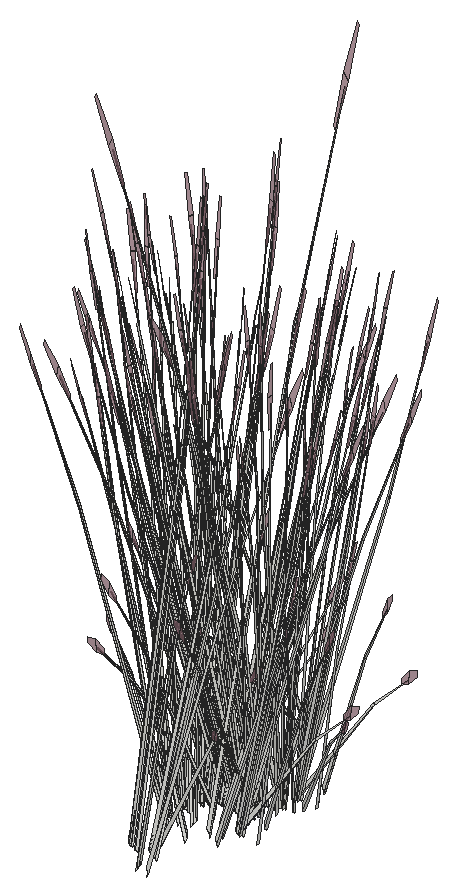
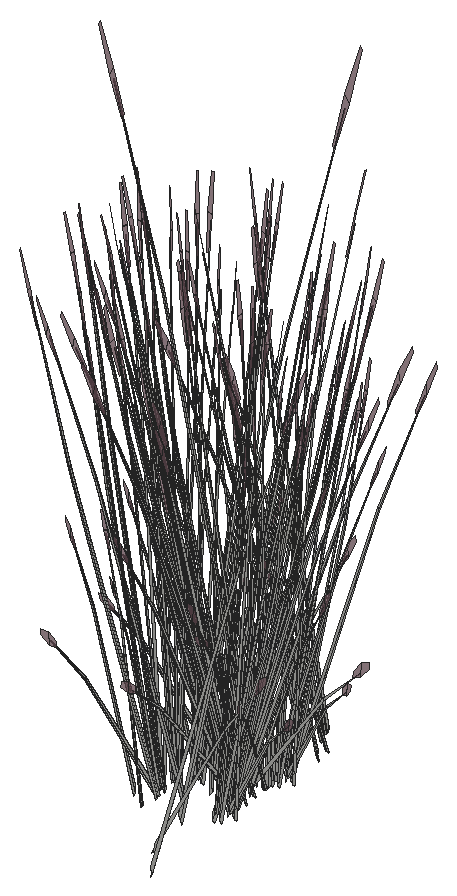
# SketchUp Ruby script. Lengths in inches.
U = 1.inch
M = Sketchup.active_model
def pt(a) = Geom::Point3d.new(a.map { |v| v * U })
def face(e, loops, mat)
  f = e.add_face(loops[0].map { |a| pt(a) })
  loops[1..].each { |l| e.add_face(l.map { |a| pt(a) }).erase! }
  f.material = f.back_material = mat if mat
  f
end
# faces: each face lists its corners as indices into pts; further lists are holes
def faces(e, pts, list, mat = nil) = list.each { |f| face(e, (f[0].is_a?(Array) ? f : [f]).map { |l| l.map { |i| pts[i] } }, mat) }
# xy, xz, yz: faces in a plane at the given z, y or x. An outline is a flat list of corners, or four numbers for a rectangle; further outlines are holes
def ring(l) = l.size == 4 ? [[l[0], l[1]], [l[2], l[1]], [l[2], l[3]], [l[0], l[3]]] : l.each_slice(2).to_a
def flat(e, list, mat, &to3) = list.each { |f| face(e, (f[0].is_a?(Array) ? f : [f]).map { |l| ring(l).map { |u, v| to3.(u, v) } }, mat) }
def xy(e, z, list, mat = nil) = flat(e, list, mat) { |x, y| [x, y, z] }
def xz(e, y, list, mat = nil) = flat(e, list, mat) { |x, z| [x, y, z] }
def yz(e, x, list, mat = nil) = flat(e, list, mat) { |y, z| [x, y, z] }
def lines(e, pts, list) = list.each { |a, b| e.add_line(pt(pts[a]), pt(pts[b])) }
# prism: a flat outline (further loops are holes) pulled along v
def prism(e, loops, v, mat = nil)
  f = face(e, loops, mat); d = Geom::Vector3d.new(v.map { |x| x * U })
  f.pushpull(f.normal.samedirection?(d) ? d.length : -d.length)
end
def box(e, o, s, mat = nil) = prism(e, [[o, [o[0] + s[0], o[1], o[2]], [o[0] + s[0], o[1] + s[1], o[2]], [o[0], o[1] + s[1], o[2]]]], [0, 0, s[2]], mat)
def at(x, y, z, deg = 0) = Geom::Transformation.translation(pt([x, y, z])) * Geom::Transformation.rotation(ORIGIN, Z_AXIS, deg.degrees)
def axes(o, x, y, z) = Geom::Transformation.new([*x, 0, *y, 0, *z, 0, *pt(o).to_a, 1])
def part(name) = M.definitions.add(name)
# library, detail: a bought-in or finely detailed component or shape, given as its bounding box
def library(name, o, s) = part(name).tap { |d| box(d.entities, o, s) }
def detail(e, o, s) = box(e.add_group.entities, o, s)
def put(e, d, t, mat = nil) = e.add_instance(d, t).tap { |i| i.material = mat if mat }
def group(e, t, mat = nil) = e.add_group.tap { |g| g.transformation = t; g.material = mat if mat }.entities
root = M.entities
M.materials.add("LightPink_Translucent").color = [144, 107, 117]
M.materials["LightPink_Translucent"].alpha = 0.75
c1 = part("blade")
p = [[2.15,0.21,22],[0,0.17,0],[0.09,0.45,0],[2.18,0.31,22],[2.29,0.31,22],[0.38,0.45,0],
  [2.48,0.24,33],[2.49,0.24,33],[2.48,0.22,33]]
faces(c1.entities,p,[[0,1,2,3],[4,5,2,3],[6,3,4,7],[8,0,3,6]])
c2 = part("seeds")
p = [[0.3,-0.1,1.38],[-0.01,-0.03,1.59],[-0.01,-0.03,0.03],[0.14,-0.07,-0.07],[0.29,-0.03,3],[0.15,0.01,3.11]]
faces(c2.entities,p,[[0,1,2,3],[1,0,4,5]],"LightPink_Translucent")
c3 = part("blade with seeds")
put(c3.entities,c1,at(0,0,0))
put(c3.entities,c2,axes([2.4,0.25,30.99],[1.5799,-0.05474,1.17369],[-0.12525,1.92788,0.29478],[-0.07173,-0.02425,1.56792]))
put(root,c3,axes([427.25,383.22,153.27],[0.16998,-0.01068,1.44779],[-0.11276,0.46299,0.11706],[-0.24224,-0.02864,0.61892]))
put(root,c3,axes([427.82,379.59,154.56],[0.45039,0.02337,-0.11403],[-0.01231,0.44247,-0.63292],[-0.03129,0.17041,0.9617]))
put(root,c3,axes([428.66,380.08,154.25],[0.40102,-0.2196,-0.10273],[0.19707,0.38974,-0.57019],[0.05291,0.16424,0.8664]))
put(root,c3,axes([430.17,387.07,154.21],[0.01066,-0.43628,-0.60019],[0.44902,0.0293,0.07243],[0.04739,-0.18483,0.84903]))
put(root,c3,axes([430.8,384.19,154.21],[0.3601,-0.20831,-0.60019],[0.20068,0.4288,0.07243],[0.17399,-0.04871,0.84903]))
put(root,c3,axes([428.13,379.76,154.23],[0.29336,0.31691,-0.47917],[-0.3099,0.27755,-0.37115],[-0.04464,0.16102,0.91684]))
put(root,c3,axes([430.79,386.39,153.98],[-0.00396,-0.09387,1.47793],[-0.33411,-0.2713,-0.23373],[0.05166,-0.16446,0.11853]))
put(root,c3,axes([429.39,386.37,153.82],[0.12355,-0.36271,-0.29918],[0.36044,0.10579,0.38624],[-0.03305,-0.14603,0.73904]))
put(root,c3,axes([429.66,386.85,153.27],[-0.0763,0.16212,1.44779],[-0.3201,-0.3355,0.11706],[0.1444,-0.2091,0.61892]))
put(root,c3,axes([430.7,386.05,153.98],[-0.04162,0.03603,1.49853],[-0.40776,-0.12155,-0.1416],[-0.01476,-0.15722,0.26519]))
put(root,c3,axes([429,380.0625,153.95],[0.40284,0.11824,-0.43168],[-0.13808,0.40538,-0.33437],[0.03694,0.16321,0.82598]))
put(root,c3,axes([429.23,379.23,153.27],[-0.09368,-0.15143,1.44779],[0.43286,-0.12749,0.11706],[0.09783,0.23774,0.61892]))
put(root,c3,axes([429.21,386.62,153.95],[-0.40284,-0.11824,-0.43168],[0.13808,-0.40538,-0.33437],[-0.03694,-0.16321,0.82598]))
put(root,c3,axes([427.18,383.57,154],[0.11578,-0.43006,0.40553],[0.38064,0.14706,0.33437],[-0.14969,0.02584,0.83914]))
put(root,c3,axes([428.82,380.3125,153.82],[-0.12355,0.36271,-0.29918],[-0.36044,-0.10579,0.38624],[0.03305,0.14603,0.73904]))
put(root,c3,axes([430.08,386.92,153.95],[-0.29336,-0.31691,-0.43168],[0.3099,-0.27755,-0.33437],[0.04464,-0.16102,0.82598]))
put(root,c3,axes([427.15,383.46,154],[-0.15051,-0.3216,0.05432],[0.27447,-0.15741,0.42765],[-0.12099,0.03106,0.65209]))
put(root,c3,axes([428.04,379.61,154.51],[-0.01066,0.43628,-0.66621],[-0.44902,-0.0293,0.0804],[-0.04739,0.18483,0.94242]))
put(root,c3,axes([428.49,385.36,153.98],[-0.00765,0.05653,1.49853],[-0.37706,0.20517,-0.1416],[-0.11096,-0.10488,0.26519]))
put(root,c3,axes([426.87,380.76,153.98],[0.04649,-0.02848,1.49853],[0.38427,0.18941,-0.1416],[-0.00903,0.15771,0.26519]))
put(root,c3,axes([428.46,379.3,153.27],[-0.01003,-0.18103,1.44779],[0.43473,0.12009,0.11706],[-0.02689,0.25798,0.61892]))
put(root,c3,axes([429.43,386.45,154],[0.4038,0.12331,0.40553],[-0.13808,0.40538,0.33437],[-0.02427,-0.15942,0.83914]))
put(root,c3,axes([429.55,386.6,154.25],[-0.40102,0.2196,-0.10273],[-0.19707,-0.38974,-0.57019],[-0.05291,-0.16424,0.8664]))
put(root,c3,axes([431.1,384.23,153.82],[0.34057,0.13158,-0.29918],[-0.09933,0.38387,0.38624],[0.13712,-0.0352,0.73904]))
put(root,c3,axes([430.38,387.09,154.25],[-0.45039,-0.02337,-0.10273],[0.01231,-0.44247,-0.57019],[0.03129,-0.17041,0.8664]))
put(root,c3,axes([430.35,386.81,153.82],[0.27728,-0.24833,-0.29918],[0.26248,0.28355,0.38624],[0.03994,-0.14407,0.73904]))
put(root,c3,axes([429.54,386.42,154],[0.30197,-0.1603,0.05432],[0.1478,0.29231,0.42765],[-0.02916,-0.12885,0.65209]))
put(root,c3,axes([428.47,386.8,154.21],[-0.34944,-0.22798,-0.60019],[0.24834,-0.39949,0.07243],[-0.1266,-0.13612,0.84903]))
put(root,c3,axes([428.85,379.99,154.21],[0.19559,0.38351,-0.60019],[-0.40262,0.21373,0.07243],[0.04574,0.1853,0.84903]))
put(root,c3,axes([428.35,386.5,153.82],[-0.06329,-0.37991,-0.29918],[0.36182,-0.10032,0.38624],[-0.09718,-0.10887,0.73904]))
put(root,c3,axes([427.1,383.62,153.82],[-0.34057,-0.13158,-0.29918],[0.09933,-0.38387,0.38624],[-0.13712,0.0352,0.73904]))
put(root,c3,axes([428.5625,380.95,153.98],[0.05195,0.07595,1.47793],[0.41921,0.02984,-0.23373],[0.04216,0.1675,0.11853]))
put(root,c3,axes([430.18,383.76,153.27],[-0.16998,0.01068,1.44779],[0.11276,-0.46299,0.11706],[0.24224,0.02864,0.61892]))
put(root,c3,axes([431.05,384.4,154],[0.15051,0.3216,0.05432],[-0.27447,0.15741,0.42765],[0.12099,-0.03106,0.65209]))
put(root,c3,axes([428.51,386.47,154],[0.18625,-0.29962,0.05432],[0.26523,0.17444,0.42765],[-0.08575,-0.09606,0.65209]))
put(root,c3,axes([431.03,384.28,154],[-0.11578,0.43006,0.40553],[-0.38064,-0.14706,0.33437],[0.14969,-0.02584,0.83914]))
put(root,c3,axes([427.57,387.05,153.27],[0.15222,0.08126,1.44779],[-0.31502,0.34091,0.11706],[-0.19634,-0.15379,0.61892]))
put(root,c3,axes([427.89,380.23,152.84],[0.009,-0.24349,1.30391],[0.40497,0.12861,0.18019],[-0.03509,0.2595,0.61571]))
put(root,c3,axes([428.31,386.8125,153.95],[-0.40438,0.11212,-0.43168],[-0.07074,-0.4246,-0.33437],[-0.10862,-0.12168,0.82598]))
put(root,c3,axes([430.35,386.9,154],[0.29182,0.32181,0.40553],[-0.3099,0.27755,0.33437],[0.05383,-0.15098,0.83914]))
put(root,c3,axes([428.14,383.56,152.82],[0.11649,-0.06823,1.49584],[0.04017,0.47639,0.11706],[-0.25231,0.06321,0.53462]))
put(root,c3,axes([428.59,386.43,154.59],[-0.2735,0.45217,-0.11506],[-0.39608,-0.2605,-0.63862],[-0.13768,-0.12775,0.97037]))
put(root,c3,axes([430.46,386.93,154],[0.33677,0.02198,0.05432],[-0.00923,0.33185,0.42765],[0.03524,-0.12712,0.65209]))
put(root,c3,axes([430.7,387.83,154.21],[0.21406,-0.37215,-0.60019],[0.37511,0.26448,0.07243],[0.12781,-0.13483,0.84903]))
put(root,c3,axes([430.6875,387.65,153.95],[-0.10528,-0.43067,-0.43168],[0.39868,-0.07534,-0.33437],[0.11425,-0.11568,0.82598]))
put(root,c3,axes([431.71,385.67,153.98],[-0.03706,-0.04129,1.49853],[0.08106,-0.44261,-0.1416],[0.14596,-0.02828,0.26519]))
put(root,c3,axes([426.89,383.88,153.98],[-0.06692,0.06124,1.47793],[0.00569,0.44742,-0.23373],[-0.15339,0.05818,0.11853]))
put(root,c3,axes([427.34,383.82,153.95],[-0.11102,0.42903,-0.43168],[-0.38064,-0.14706,-0.33437],[-0.15325,0.03934,0.82598]))
put(root,c3,axes([427.32,383.45,154.25],[0.20619,0.42709,-0.10273],[-0.36595,0.20988,-0.57019],[-0.15422,0.05635,0.8664]))
put(root,c3,axes([427.54,386.3,153.98],[-0.08817,-0.00333,1.47793],[-0.28072,0.33293,-0.23373],[-0.14978,-0.06803,0.11853]))
put(root,c3,axes([430.875,387.96,154.25],[-0.37908,-0.26007,-0.10273],[0.21839,-0.37663,-0.57019],[0.1071,-0.13092,0.8664]))
put(root,c3,axes([431.39,385.3,153.32],[-0.07843,-0.39649,-0.0295],[0.37072,-0.09115,-0.13375],[0.07742,0.02514,0.44114]))
put(root,c3,axes([430.43,385.29,154.25],[0.02194,-0.47967,-0.10273],[0.41546,0.01311,-0.57019],[0.16001,0.03332,0.8664]))
put(root,c3,axes([429.31,389.38,152.81],[0.35414,0.19019,1.27785],[-0.34693,0.40974,0.50532],[-0.1554,-0.24285,1.07126]))
put(root,c3,axes([431.81,387.85,153.98],[-0.05353,-0.00358,1.49853],[-0.22227,-0.38383,-0.1416],[0.08926,-0.1262,0.26519]))
put(root,c3,axes([430.79,385,153.98],[0.08791,-0.00798,1.47793],[0.24113,-0.36643,-0.23373],[0.15637,0.04837,0.11853]))
put(root,c3,axes([430.98,387.7,153.82],[0.35672,-0.06741,-0.29918],[0.09419,0.38534,0.38624],[0.10222,-0.1035,0.73904]))
put(root,c3,axes([427.27,384.65,154],[-0.10163,-0.43409,0.40553],[0.39868,-0.07534,0.33437],[-0.1175,0.10209,0.83914]))
put(root,c3,axes([427.63,387.06,154],[0.02064,-0.35866,0.05432],[0.3116,0.00983,0.42765],[-0.11936,-0.03753,0.65209]))
put(root,c3,axes([427.19,384.5625,154],[-0.28133,-0.19836,0.05432],[0.16379,-0.28248,0.42765],[-0.0902,0.09132,0.65209]))
put(root,c3,axes([427.32,384.04,153.27],[0.14219,-0.09977,1.44779],[0.11971,0.461,0.11706],[-0.22323,0.10419,0.61892]))
put(root,c3,axes([427.51,387.17,153.82],[-0.23317,-0.29531,-0.29918],[0.26625,-0.27955,0.38624],[-0.13527,-0.04253,0.73904]))
put(root,c3,axes([430.45,385.0625,154.21],[0.40965,0.01136,-0.60019],[-0.02751,0.47821,0.07243],[0.17355,0.05047,0.84903]))
put(root,c3,axes([427.76,387.37,154.21],[-0.40965,-0.01136,-0.60019],[0.02751,-0.47821,0.07243],[-0.17355,-0.05047,0.84903]))
put(root,c3,axes([426.14,384.33,153.98],[0.0523,0.01265,1.49853],[0.16179,0.41674,-0.1416],[-0.10706,0.10938,0.26519]))
put(root,c3,axes([430.69,385.26,153.82],[0.23317,0.29531,-0.29918],[-0.26625,0.27955,0.38624],[0.13527,0.04253,0.73904]))
put(root,c3,axes([431.01,387.86,154],[0.28133,0.19836,0.05432],[-0.16379,0.28248,0.42765],[0.0902,-0.09132,0.65209]))
put(root,c3,axes([430.57,385.37,154],[-0.02064,0.35866,0.05432],[-0.3116,-0.00983,0.42765],[0.11936,0.03753,0.65209]))
put(root,c3,axes([430.93,387.78,154],[0.10163,0.43409,0.40553],[-0.39868,0.07534,0.33437],[0.1175,-0.10209,0.83914]))
put(root,c3,axes([432.01,388.31,153.98],[0.05687,-0.07184,1.47793],[-0.07279,-0.44069,-0.23373],[0.14268,-0.08356,0.11853]))
put(root,c3,axes([427.23,384.73,153.82],[-0.35672,0.06741,-0.29918],[-0.09419,-0.38534,0.38624],[-0.10222,0.1035,0.73904]))
put(root,c3,axes([430.6,385.26,154],[-0.30217,0.31079,0.40553],[-0.2606,-0.33005,0.33437],[0.14177,0.05733,0.83914]))
put(root,c3,axes([427.2,386.59,153.98],[0.03038,0.04707,1.49853],[-0.14646,0.42312,-0.1416],[-0.14833,0.00306,0.26519]))
put(root,c3,axes([427.625,387.46,153.95],[-0.29757,0.31243,-0.43168],[-0.2606,-0.33005,-0.33437],[-0.15119,-0.04754,0.82598]))
put(root,c3,axes([429.86,384.5,153.27],[-0.15222,-0.08126,1.44779],[0.31502,-0.34091,0.11706],[0.19634,0.15379,0.61892]))
put(root,c3,axes([429.88,383.43,153.78],[-0.35411,-0.24507,1.16821],[0.37391,-0.38156,0.50405],[0.11425,0.22994,1.12919]))
put(root,c3,axes([427.78,387.13,154.25],[-0.02194,0.47967,-0.10273],[-0.41546,-0.01311,-0.57019],[-0.16001,-0.03332,0.8664]))
put(root,c3,axes([427.33,384.47,154.25],[0.37908,0.26007,-0.10273],[-0.21839,0.37663,-0.57019],[-0.1071,0.13092,0.8664]))
put(root,c3,axes([430.89,388.98,154.25],[-0.20619,-0.42709,-0.10273],[0.36595,-0.20988,-0.57019],[0.15422,-0.05635,0.8664]))
put(root,c3,axes([430.87,388.61,153.95],[0.11102,-0.42903,-0.43168],[0.38064,0.14706,-0.33437],[0.15325,-0.03934,0.82598]))
put(root,c3,axes([429.61,385.8125,154.25],[0.2442,-0.40372,-0.10273],[0.35364,0.23259,-0.57019],[0.12293,0.11406,0.8664]))
put(root,c3,axes([427.25,387.8,153.27],[0.16998,-0.01068,1.44779],[-0.11276,0.46299,0.11706],[-0.24224,-0.02864,0.61892]))
put(root,c3,axes([427.84,384.35,153.27],[0.10236,-0.14492,1.44779],[0.25844,0.39118,0.11706],[-0.17726,0.17814,0.61892]))
put(root,c3,axes([427.52,384.77,153.95],[0.10528,0.43067,-0.43168],[-0.39868,0.07534,-0.33437],[-0.11425,0.11568,0.82598]))
put(root,c3,axes([429.29,386.15,153.98],[0.00121,-0.0571,1.49853],[0.35119,-0.25193,-0.1416],[0.12199,0.08992,0.26519]))
put(root,c3,axes([430.8,388.77,154.21],[0.3601,-0.20831,-0.60019],[0.20068,0.4288,0.07243],[0.17399,-0.04871,0.84903]))
put(root,c3,axes([427.75,385.49,154],[-0.33677,-0.02198,0.05432],[0.00923,-0.33185,0.42765],[-0.03524,0.12712,0.65209]))
put(root,c3,axes([427.85,385.52,154],[-0.29182,-0.32181,0.40553],[0.3099,-0.27755,0.33437],[-0.05383,0.15098,0.83914]))
put(root,c3,axes([429.9,385.61,153.95],[0.40438,-0.11212,-0.43168],[0.07074,0.4246,-0.33437],[0.10862,0.12168,0.82598]))
put(root,c3,axes([427.18,388.15,154],[0.11578,-0.43006,0.40553],[0.38064,0.14706,0.33437],[-0.14969,0.02584,0.83914]))
put(root,c3,axes([429.7,385.96,154],[-0.18625,0.29962,0.05432],[-0.26523,-0.17444,0.42765],[0.08575,0.09606,0.65209]))
put(root,c3,axes([427.15,388.03,154],[-0.15051,-0.3216,0.05432],[0.27447,-0.15741,0.42765],[-0.12099,0.03106,0.65209]))
put(root,c3,axes([429.78,385.88,154],[-0.4076,0.10824,0.40553],[-0.07074,-0.4246,0.33437],[0.09586,0.12514,0.83914]))
put(root,c3,axes([427.77,384.71,153.27],[0.0763,-0.16212,1.44779],[0.3201,0.3355,0.11706],[-0.1444,0.2091,0.61892]))
put(root,c3,axes([431.1,388.8,153.82],[0.34057,0.13158,-0.29918],[-0.09933,0.38387,0.38624],[0.13712,-0.0352,0.73904]))
put(root,c3,axes([428.66,386.01,154],[-0.30197,0.1603,0.05432],[-0.1478,-0.29231,0.42765],[0.02916,0.12885,0.65209]))
put(root,c3,axes([427.85,385.62,153.82],[-0.27728,0.24833,-0.29918],[-0.26248,-0.28355,0.38624],[-0.03994,0.14407,0.73904]))
put(root,c3,axes([426.9,385.55,153.98],[-0.01019,0.09334,1.47793],[0.28908,0.3247,-0.23373],[-0.07568,0.15355,0.11853]))
put(root,c3,axes([427.82,385.34,154.56],[0.45039,0.02337,-0.11403],[-0.01231,0.44247,-0.63292],[-0.03129,0.17041,0.9617]))
put(root,c3,axes([427.1,388.19,153.82],[-0.34057,-0.13158,-0.29918],[0.09933,-0.38387,0.38624],[-0.13712,0.0352,0.73904]))
put(root,c3,axes([428.66,385.83,154.25],[0.40102,-0.2196,-0.10273],[0.19707,0.38974,-0.57019],[0.05291,0.16424,0.8664]))
put(root,c3,axes([430.18,388.33,153.27],[-0.16998,0.01068,1.44779],[0.11276,-0.46299,0.11706],[0.24224,0.02864,0.61892]))
put(root,c3,axes([431.05,388.97,154],[0.15051,0.3216,0.05432],[-0.27447,0.15741,0.42765],[0.12099,-0.03106,0.65209]))
put(root,c3,axes([428.13,385.5,154.23],[0.29336,0.31691,-0.47917],[-0.3099,0.27755,-0.37115],[-0.04464,0.16102,0.91684]))
put(root,c3,axes([431.03,388.85,154],[-0.11578,0.43006,0.40553],[-0.38064,-0.14706,0.33437],[0.14969,-0.02584,0.83914]))
put(root,c3,axes([429,385.8125,153.95],[0.40284,0.11824,-0.43168],[-0.13808,0.40538,-0.33437],[0.03694,0.16321,0.82598]))
put(root,c3,axes([429.23,384.97,153.27],[-0.09368,-0.15143,1.44779],[0.43286,-0.12749,0.11706],[0.09783,0.23774,0.61892]))
put(root,c3,axes([428.82,386.06,153.82],[-0.12355,0.36271,-0.29918],[-0.36044,-0.10579,0.38624],[0.03305,0.14603,0.73904]))
put(root,c3,axes([428.14,388.13,152.82],[0.11649,-0.06823,1.49584],[0.04017,0.47639,0.11706],[-0.25231,0.06321,0.53462]))
put(root,c3,axes([428.04,385.36,154.51],[-0.01066,0.43628,-0.66621],[-0.44902,-0.0293,0.0804],[-0.04739,0.18483,0.94242]))
put(root,c3,axes([426.87,386.5,153.98],[0.04649,-0.02848,1.49853],[0.38427,0.18941,-0.1416],[-0.00903,0.15771,0.26519]))
put(root,c3,axes([428.46,385.05,153.27],[-0.01003,-0.18103,1.44779],[0.43473,0.12009,0.11706],[-0.02689,0.25798,0.61892]))
put(root,c3,axes([431.71,390.24,153.98],[-0.03706,-0.04129,1.49853],[0.08106,-0.44261,-0.1416],[0.14596,-0.02828,0.26519]))
put(root,c3,axes([426.89,388.45,153.98],[-0.06692,0.06124,1.47793],[0.00569,0.44742,-0.23373],[-0.15339,0.05818,0.11853]))
put(root,c3,axes([428.85,385.73,154.21],[0.19559,0.38351,-0.60019],[-0.40262,0.21373,0.07243],[0.04574,0.1853,0.84903]))
put(root,c3,axes([427.34,388.39,153.95],[-0.11102,0.42903,-0.43168],[-0.38064,-0.14706,-0.33437],[-0.15325,0.03934,0.82598]))
put(root,c3,axes([427.32,388.02,154.25],[0.20619,0.42709,-0.10273],[-0.36595,0.20988,-0.57019],[-0.15422,0.05635,0.8664]))
put(root,c3,axes([431.39,389.875,153.32],[-0.07843,-0.39649,-0.0295],[0.37072,-0.09115,-0.13375],[0.07742,0.02514,0.44114]))
put(root,c3,axes([430.43,389.86,154.25],[0.02194,-0.47967,-0.10273],[0.41546,0.01311,-0.57019],[0.16001,0.03332,0.8664]))
put(root,c3,axes([428.5625,386.7,153.98],[0.05195,0.07595,1.47793],[0.41921,0.02984,-0.23373],[0.04216,0.1675,0.11853]))
put(root,c3,axes([427.89,385.97,152.84],[0.009,-0.24349,1.30391],[0.40497,0.12861,0.18019],[-0.03509,0.2595,0.61571]))
put(root,c3,axes([430.79,389.58,153.98],[0.08791,-0.00798,1.47793],[0.24113,-0.36643,-0.23373],[0.15637,0.04837,0.11853]))
put(root,c3,axes([427.27,389.22,154],[-0.10163,-0.43409,0.40553],[0.39868,-0.07534,0.33437],[-0.1175,0.10209,0.83914]))
put(root,c3,axes([427.19,389.13,154],[-0.28133,-0.19836,0.05432],[0.16379,-0.28248,0.42765],[-0.0902,0.09132,0.65209]))
put(root,c3,axes([427.32,388.61,153.27],[0.14219,-0.09977,1.44779],[0.11971,0.461,0.11706],[-0.22323,0.10419,0.61892]))
put(root,c3,axes([430.45,389.63,154.21],[0.40965,0.01136,-0.60019],[-0.02751,0.47821,0.07243],[0.17355,0.05047,0.84903]))
put(root,c3,axes([426.84,395.01,153.27],[0.09368,0.15143,1.44779],[-0.43286,0.12749,0.11706],[-0.09783,-0.23774,0.61892]))
put(root,c3,axes([426.14,388.9,153.98],[0.0523,0.01265,1.49853],[0.16179,0.41674,-0.1416],[-0.10706,0.10938,0.26519]))
put(root,c3,axes([427.56,394,153.98],[-0.06268,-0.06613,1.47793],[-0.4183,0.04193,-0.23373],[-0.06676,-0.15817,0.11853]))
